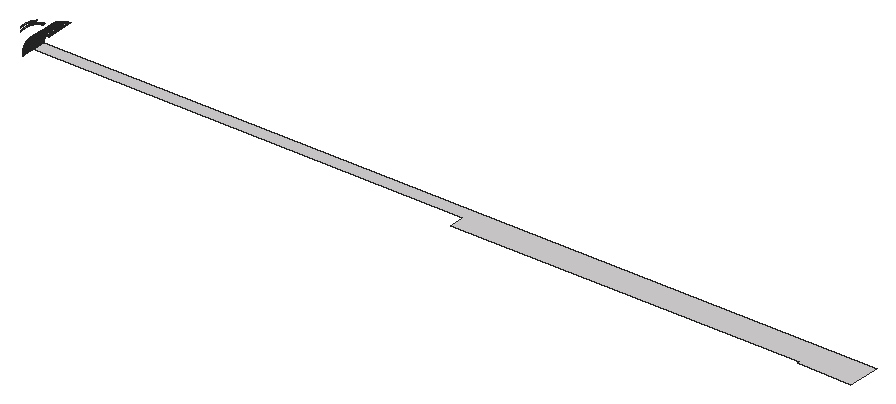
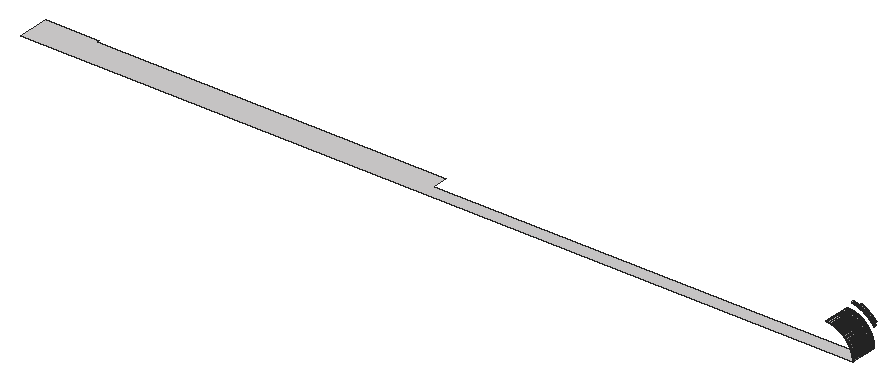
# SketchUp Ruby script. Lengths in inches.
U = 1.inch
M = Sketchup.active_model
def pt(a) = Geom::Point3d.new(a.map { |v| v * U })
def face(e, loops, mat)
  f = e.add_face(loops[0].map { |a| pt(a) })
  loops[1..].each { |l| e.add_face(l.map { |a| pt(a) }).erase! }
  f.material = f.back_material = mat if mat
  f
end
# faces: each face lists its corners as indices into pts; further lists are holes
def faces(e, pts, list, mat = nil) = list.each { |f| face(e, (f[0].is_a?(Array) ? f : [f]).map { |l| l.map { |i| pts[i] } }, mat) }
# xy, xz, yz: faces in a plane at the given z, y or x. An outline is a flat list of corners, or four numbers for a rectangle; further outlines are holes
def ring(l) = l.size == 4 ? [[l[0], l[1]], [l[2], l[1]], [l[2], l[3]], [l[0], l[3]]] : l.each_slice(2).to_a
def flat(e, list, mat, &to3) = list.each { |f| face(e, (f[0].is_a?(Array) ? f : [f]).map { |l| ring(l).map { |u, v| to3.(u, v) } }, mat) }
def xy(e, z, list, mat = nil) = flat(e, list, mat) { |x, y| [x, y, z] }
def xz(e, y, list, mat = nil) = flat(e, list, mat) { |x, z| [x, y, z] }
def yz(e, x, list, mat = nil) = flat(e, list, mat) { |y, z| [x, y, z] }
def lines(e, pts, list) = list.each { |a, b| e.add_line(pt(pts[a]), pt(pts[b])) }
# prism: a flat outline (further loops are holes) pulled along v
def prism(e, loops, v, mat = nil)
  f = face(e, loops, mat); d = Geom::Vector3d.new(v.map { |x| x * U })
  f.pushpull(f.normal.samedirection?(d) ? d.length : -d.length)
end
def box(e, o, s, mat = nil) = prism(e, [[o, [o[0] + s[0], o[1], o[2]], [o[0] + s[0], o[1] + s[1], o[2]], [o[0], o[1] + s[1], o[2]]]], [0, 0, s[2]], mat)
def at(x, y, z, deg = 0) = Geom::Transformation.translation(pt([x, y, z])) * Geom::Transformation.rotation(ORIGIN, Z_AXIS, deg.degrees)
def axes(o, x, y, z) = Geom::Transformation.new([*x, 0, *y, 0, *z, 0, *pt(o).to_a, 1])
def part(name) = M.definitions.add(name)
# library, detail: a bought-in or finely detailed component or shape, given as its bounding box
def library(name, o, s) = part(name).tap { |d| box(d.entities, o, s) }
def detail(e, o, s) = box(e.add_group.entities, o, s)
def put(e, d, t, mat = nil) = e.add_instance(d, t).tap { |i| i.material = mat if mat }
def group(e, t, mat = nil) = e.add_group.tap { |g| g.transformation = t; g.material = mat if mat }.entities
root = M.entities
M.materials.add("[Quartz Light Brown]").color = [215, 212, 212]
xy(root,84,[[372,36,396,36,396,50,24,50,24,44,216,44,216,37,372,37]],"[Quartz Light Brown]")
xy(root,95.96,[[34.96,38,35.06,50]],"[Quartz Light Brown]")
xy(root,95.98,[[35.25,38,35.34,50]],"[Quartz Light Brown]")
xy(root,95.99,[[35.43,38,35.53,50],[35.53,38,35.625,50]],"[Quartz Light Brown]")
xy(root,96,[[35.72,38,35.8125,50],[35.8125,38,35.91,50],[35.91,38,36,50]],"[Quartz Light Brown]")
yz(root,24,[[38,84,50,84.09],[38,84.09,50,84.1875],[38,84.1875,50,84.28]],"[Quartz Light Brown]")
yz(root,24.01,[[38,84.375,50,84.47],[38,84.47,50,84.57]],"[Quartz Light Brown]")
yz(root,24.02,[[38,84.66,50,84.75]],"[Quartz Light Brown]")
yz(root,24.04,[[38,84.94,50,85.04]],"[Quartz Light Brown]")
p = [[24.01,38,84.375],[24,38,84.28],[24,50,84.28],[24.01,50,84.375],[24.02,38,84.66],[24.01,38,84.57],
  [24.01,50,84.57],[24.02,50,84.66],[24.03,38,84.85],[24.02,38,84.75],[24.02,50,84.75],[24.03,50,84.85],
  [24.04,38,84.94],[24.04,50,84.94],[24.05,38,85.13],[24.04,38,85.04],[24.04,50,85.04],[24.05,50,85.13],
  [24.0625,38,85.22],[24.0625,50,85.22],[24.07,38,85.32],[24.07,50,85.32],[24.08,38,85.41],[24.08,50,85.41],
  [24.09,38,85.5],[24.09,50,85.5],[24.11,38,85.6],[24.11,50,85.6],[24.12,38,85.69],[24.12,50,85.69],
  [24.13,38,85.78],[24.13,50,85.78],[24.15,38,85.88],[24.15,50,85.88],[24.16,38,85.97],[24.16,50,85.97],
  [24.18,38,86.0625],[24.18,50,86.0625],[24.2,38,86.16],[24.2,50,86.16],[24.21,38,86.25],[24.21,50,86.25],
  [24.23,38,86.34],[24.23,50,86.34],[24.25,38,86.43],[24.25,50,86.43],[24.27,38,86.53],[24.27,50,86.53],
  [24.29,38,86.62],[24.29,50,86.62],[24.31,38,86.71],[24.31,50,86.71],[24.33,38,86.8],[24.33,50,86.8],
  [24.35,38,86.89],[24.35,50,86.89],[24.38,38,86.98],[24.38,50,86.98],[24.4,38,87.08],[24.4,50,87.08],
  [24.43,38,87.17],[24.43,50,87.17],[24.45,38,87.26],[24.45,50,87.26],[24.48,38,87.35],[24.48,50,87.35],
  [24.5,38,87.4375],[24.5,50,87.4375],[24.53,38,87.53],[24.53,50,87.53],[24.56,38,87.62],[24.56,50,87.62],
  [24.59,38,87.71],[24.59,50,87.71],[24.62,38,87.8],[24.62,50,87.8],[24.65,38,87.89],[24.65,50,87.89],
  [24.68,38,87.98],[24.68,50,87.98],[24.71,38,88.06],[24.71,50,88.06],[24.74,38,88.15],[24.74,50,88.15],
  [24.77,38,88.24],[24.77,50,88.24],[24.81,38,88.33],[24.81,50,88.33],[24.84,38,88.42],[24.84,50,88.42],
  [24.88,38,88.5],[24.88,50,88.5],[24.91,38,88.59],[24.91,50,88.59],[24.95,38,88.68],[24.95,50,88.68],
  [24.99,38,88.77],[24.99,50,88.77],[25.02,38,88.85],[25.02,50,88.85],[25.0625,38,88.9375],[25.0625,50,88.9375],
  [25.1,38,89.02],[25.1,50,89.02],[25.14,38,89.11],[25.14,50,89.11],[25.18,38,89.19],[25.18,50,89.19],
  [25.22,38,89.28],[25.22,50,89.28],[25.27,38,89.36],[25.27,50,89.36],[25.31,38,89.45],[25.31,50,89.45],
  [25.35,38,89.53],[25.35,50,89.53],[25.39,38,89.62],[25.39,50,89.62],[25.4375,38,89.7],[25.4375,50,89.7],
  [25.48,38,89.78],[25.48,50,89.78],[25.53,38,89.86],[25.53,50,89.86],[25.58,38,89.95],[25.58,50,89.95],
  [25.625,38,90.03],[25.625,50,90.03],[25.67,38,90.11],[25.67,50,90.11],[25.72,38,90.1875],[25.72,50,90.1875],
  [25.77,38,90.27],[25.77,50,90.27],[25.82,38,90.35],[25.82,50,90.35],[25.87,38,90.43],[25.87,50,90.43],
  [25.92,38,90.51],[25.92,50,90.51],[25.97,38,90.59],[25.97,50,90.59],[26.02,38,90.67],[26.02,50,90.67],
  [26.08,38,90.75],[26.08,50,90.75],[26.13,38,90.82],[26.13,50,90.82],[26.18,38,90.9],[26.18,50,90.9],
  [26.24,38,90.98],[26.24,50,90.98],[26.29,38,91.05],[26.29,50,91.05],[26.35,38,91.13],[26.35,50,91.13],
  [26.4,38,91.21],[26.4,50,91.21],[26.46,38,91.28],[26.46,50,91.28],[26.52,38,91.35],[26.52,50,91.35],
  [26.58,38,91.43],[26.58,50,91.43],[26.63,38,91.5],[26.63,50,91.5],[26.69,38,91.58],[26.69,50,91.58],
  [26.75,38,91.65],[26.75,50,91.65],[26.8125,38,91.72],[26.8125,50,91.72],[26.875,38,91.79],[26.875,50,91.79],
  [26.9375,38,91.86],[26.9375,50,91.86],[27,38,91.9375],[27,50,91.9375],[27.0625,38,92.01],[27.0625,50,92.01],
  [27.125,38,92.08],[27.125,50,92.08],[27.1875,38,92.15],[27.1875,50,92.15],[27.25,38,92.21],[27.25,50,92.21],
  [27.32,38,92.28],[27.32,50,92.28],[27.38,38,92.35],[27.38,50,92.35],[27.45,38,92.42],[27.45,50,92.42],
  [27.51,38,92.49],[27.51,50,92.49],[27.58,38,92.55],[27.58,50,92.55],[27.65,38,92.62],[27.65,50,92.62],
  [27.72,38,92.68],[27.72,50,92.68],[27.79,38,92.75],[27.79,50,92.75],[27.85,38,92.8125],[27.85,50,92.8125],
  [27.92,38,92.875],[27.92,50,92.875],[27.99,38,92.9375],[27.99,50,92.9375],[28.0625,38,93],[28.0625,50,93],
  [28.14,38,93.0625],[28.14,50,93.0625],[28.21,38,93.125],[28.21,50,93.125],[28.28,38,93.1875],[28.28,50,93.1875],
  [28.35,38,93.25],[28.35,50,93.25],[28.42,38,93.31],[28.42,50,93.31],[28.5,38,93.37],[28.5,50,93.37],
  [23.06,39,93.4],[23.06,38,93.4],[23.13,38,93.51],[23.13,39,93.51],[28.57,38,93.42],[28.57,50,93.42],
  [28.65,38,93.48],[28.65,50,93.48],[23.21,38,93.61],[23.21,39,93.61],[28.72,38,93.54],[28.72,50,93.54],
  [28.79,38,93.6],[28.79,50,93.6],[23.28,38,93.71],[23.28,39,93.71],[28.87,38,93.65],[28.87,50,93.65],
  [23.36,38,93.81],[23.36,39,93.81],[28.95,38,93.71],[28.95,50,93.71],[29.02,38,93.76],[29.02,50,93.76],
  [23.44,38,93.91],[23.44,39,93.91],[29.1,38,93.82],[29.1,50,93.82],[29.18,38,93.87],[29.18,50,93.87],
  [23.51,38,94],[23.51,39,94],[29.25,38,93.92],[29.25,50,93.92],[29.33,38,93.98],[29.33,50,93.98],
  [23.59,38,94.1],[23.59,39,94.1],[29.41,38,94.03],[29.41,50,94.03],[29.49,38,94.08],[29.49,50,94.08],
  [23.67,38,94.2],[23.67,39,94.2],[29.57,38,94.13],[29.57,50,94.13],[29.65,38,94.18],[29.65,50,94.18],
  [23.75,38,94.3],[23.75,39,94.3],[29.73,38,94.23],[29.73,50,94.23],[29.8125,38,94.28],[29.8125,50,94.28],
  [23.83,38,94.39],[23.83,39,94.39],[29.89,38,94.33],[29.89,50,94.33],[29.97,38,94.375],[29.97,50,94.375],
  [23.92,38,94.49],[23.92,39,94.49],[30.05,38,94.42],[30.05,50,94.42],[30.14,38,94.47],[30.14,50,94.47],
  [24,38,94.58],[24,39,94.58],[30.22,38,94.52],[30.22,50,94.52],[30.3,38,94.5625],[30.3,50,94.5625],
  [24.08,38,94.67],[24.08,39,94.67],[30.38,38,94.61],[30.38,50,94.61],[30.47,38,94.65],[30.47,50,94.65],
  [30.55,38,94.69],[30.55,50,94.69],[24.17,38,94.77],[24.17,39,94.77],[30.64,38,94.73],[30.64,50,94.73],
  [30.72,38,94.78],[30.72,50,94.78],[24.25,38,94.86],[24.25,39,94.86],[30.81,38,94.82],[30.81,50,94.82],
  [30.89,38,94.86],[30.89,50,94.86],[22.99,38,94.9375],[22.99,39,94.9375],[23.07,39,95.04],[23.07,38,95.04],
  [24.34,38,94.95],[24.34,39,94.95],[30.98,38,94.9],[30.98,50,94.9],[31.0625,38,94.9375],[31.0625,50,94.9375],
  [31.15,38,94.98],[31.15,50,94.98],[23.16,39,95.14],[23.16,38,95.14],[24.42,38,95.04],[24.42,39,95.04],
  [24.51,38,95.13],[24.51,39,95.13],[31.23,38,95.01],[31.23,50,95.01],[31.32,38,95.05],[31.32,50,95.05],
  [23.25,39,95.24],[23.25,38,95.24],[24.6,38,95.22],[24.6,39,95.22],[31.41,38,95.09],[31.41,50,95.09],
  [31.5,38,95.12],[31.5,50,95.12],[31.58,38,95.16],[31.58,50,95.16],[23.34,39,95.34],[23.34,38,95.34],
  [24.6875,38,95.3125],[24.6875,39,95.3125],[31.67,38,95.19],[31.67,50,95.19],[31.76,38,95.23],[31.76,50,95.23],
  [31.85,38,95.26],[31.85,50,95.26],[23.43,39,95.44],[23.43,38,95.44],[24.78,38,95.4],[24.78,39,95.4],
  [31.94,38,95.29],[31.94,50,95.29],[32.02,38,95.32],[32.02,50,95.32],[32.11,38,95.35],[32.11,50,95.35],
  [23.52,39,95.54],[23.52,38,95.54],[24.87,38,95.49],[24.87,39,95.49],[32.2,38,95.38],[32.2,50,95.38],
  [32.29,38,95.41],[32.29,50,95.41],[32.38,38,95.44],[32.38,50,95.44],[32.47,38,95.47],[32.47,50,95.47],
  [23.61,39,95.64],[23.61,38,95.64],[24.96,38,95.58],[24.96,39,95.58],[32.5625,38,95.5],[32.5625,50,95.5],
  [32.65,38,95.52],[32.65,50,95.52],[32.74,38,95.55],[32.74,50,95.55],[32.83,38,95.57],[32.83,50,95.57],
  [23.7,39,95.73],[23.7,38,95.73],[25.05,38,95.66],[25.05,39,95.66],[32.92,38,95.6],[32.92,50,95.6],
  [33.02,38,95.62],[33.02,50,95.62],[33.11,38,95.65],[33.11,50,95.65],[33.2,38,95.67],[33.2,50,95.67],
  [23.79,39,95.83],[23.79,38,95.83],[25.14,38,95.75],[25.14,39,95.75],[25.23,38,95.83],[25.23,39,95.83],
  [33.29,38,95.69],[33.29,50,95.69],[33.38,38,95.71],[33.38,50,95.71],[33.47,38,95.73],[33.47,50,95.73],
  [33.57,38,95.75],[33.57,50,95.75],[23.89,39,95.93],[23.89,38,95.93],[25.33,38,95.92],[25.33,39,95.92],
  [33.66,38,95.77],[33.66,50,95.77],[33.75,38,95.79],[33.75,50,95.79],[33.84,38,95.8],[33.84,50,95.8],
  [33.9375,38,95.82],[33.9375,50,95.82],[34.03,38,95.84],[34.03,50,95.84],[34.12,38,95.85],[34.12,50,95.85],
  [23.98,39,96.02],[23.98,38,96.02],[25.42,38,96],[25.42,39,96],[34.22,38,95.87],[34.22,50,95.87],
  [34.31,38,95.88],[34.31,50,95.88],[34.4,38,95.89],[34.4,50,95.89],[34.5,38,95.91],[34.5,50,95.91],
  [34.59,38,95.92],[34.59,50,95.92],[34.68,38,95.93],[34.68,50,95.93],[34.78,38,95.9375],[34.78,50,95.9375],
  [34.87,38,95.95],[34.87,50,95.95],[34.96,38,95.96],[34.96,50,95.96],[24.07,39,96.11],[24.07,38,96.11],
  [25.51,38,96.08],[25.51,39,96.08],[35.15,38,95.97],[35.06,38,95.96],[35.06,50,95.96],[35.15,50,95.97],
  [35.25,38,95.98],[35.25,50,95.98],[35.43,38,95.99],[35.34,38,95.98],[35.34,50,95.98],[35.43,50,95.99],
  [35.72,38,96],[35.625,38,95.99],[35.625,50,95.99],[35.72,50,96],[24.17,39,96.21],[24.17,38,96.21],
  [25.61,38,96.17],[25.61,39,96.17],[24.27,39,96.3],[24.27,38,96.3],[25.7,38,96.25],[25.7,39,96.25],
  [25.8,38,96.33],[25.8,39,96.33],[24.36,39,96.39],[24.36,38,96.39],[25.9,38,96.41],[25.9,39,96.41],
  [24.46,39,96.48],[24.46,38,96.48],[26,38,96.49],[26,39,96.49],[24.56,39,96.57],[24.56,38,96.57],
  [26.09,38,96.56],[26.09,39,96.56],[24.66,39,96.66],[24.66,38,96.66],[26.19,38,96.64],[26.19,39,96.64],
  [26.29,38,96.72],[26.29,39,96.72],[24.76,39,96.75],[24.76,38,96.75],[26.39,38,96.79],[26.39,39,96.79],
  [24.86,39,96.84],[24.86,38,96.84],[24.96,39,96.93],[24.96,38,96.93],[26.49,38,96.87],[26.49,39,96.87],
  [25.0625,39,97.01],[25.0625,38,97.01],[26.6,38,96.94],[26.6,39,96.94],[26.7,38,97.02],[26.7,39,97.02],
  [25.16,39,97.1],[25.16,38,97.1],[26.8,38,97.09],[26.8,39,97.09],[25.27,39,97.18],[25.27,38,97.18],
  [26.9,38,97.16],[26.9,39,97.16],[25.37,39,97.27],[25.37,38,97.27],[27.01,38,97.23],[27.01,39,97.23],
  [27.11,38,97.3],[27.11,39,97.3],[25.48,39,97.35],[25.48,38,97.35],[27.22,38,97.37],[27.22,39,97.37],
  [25.58,39,97.43],[25.58,38,97.43],[25.6875,39,97.51],[25.6875,38,97.51],[27.32,38,97.44],[27.32,39,97.44],
  [27.43,38,97.51],[27.43,39,97.51],[25.79,39,97.59],[25.79,38,97.59],[27.53,38,97.58],[27.53,39,97.58],
  [25.9,39,97.67],[25.9,38,97.67],[27.64,38,97.64],[27.64,39,97.64],[27.75,38,97.71],[27.75,39,97.71],
  [26.01,39,97.75],[26.01,38,97.75],[27.86,38,97.77],[27.86,39,97.77],[26.12,39,97.83],[26.12,38,97.83],
  [26.22,39,97.91],[26.22,38,97.91],[27.96,38,97.84],[27.96,39,97.84],[28.07,38,97.9],[28.07,39,97.9],
  [26.33,39,97.98],[26.33,38,97.98],[28.18,38,97.96],[28.18,39,97.96],[26.44,39,98.06],[26.44,38,98.06],
  [28.29,38,98.02],[28.29,39,98.02],[28.4,38,98.08],[28.4,39,98.08],[26.56,39,98.13],[26.56,38,98.13],
  [26.67,39,98.21],[26.67,38,98.21],[28.51,38,98.14],[28.51,39,98.14],[28.625,38,98.2],[28.625,39,98.2],
  [26.78,39,98.28],[26.78,38,98.28],[28.74,38,98.26],[28.74,39,98.26],[26.89,39,98.35],[26.89,38,98.35],
  [28.85,38,98.3125],[28.85,39,98.3125],[28.96,38,98.37],[28.96,39,98.37],[27,39,98.42],[27,38,98.42],
  [27.12,39,98.49],[27.12,38,98.49],[29.07,38,98.42],[29.07,39,98.42],[29.1875,38,98.48],[29.1875,39,98.48],
  [27.23,39,98.5625],[27.23,38,98.5625],[29.3,38,98.53],[29.3,39,98.53],[29.42,38,98.58],[29.42,39,98.58],
  [27.35,39,98.63],[27.35,38,98.63],[27.46,39,98.7],[27.46,38,98.7],[29.53,38,98.63],[29.53,39,98.63],
  [29.65,38,98.68],[29.65,39,98.68],[27.58,39,98.77],[27.58,38,98.77],[29.76,38,98.73],[29.76,39,98.73],
  [29.88,38,98.78],[29.88,39,98.78],[27.69,39,98.83],[27.69,38,98.83],[27.81,39,98.9],[27.81,38,98.9],
  [29.99,38,98.83],[29.99,39,98.83],[30.11,38,98.875],[30.11,39,98.875],[27.93,39,98.96],[27.93,38,98.96],
  [30.23,38,98.92],[30.23,39,98.92],[30.34,38,98.97],[30.34,39,98.97],[28.05,39,99.02],[28.05,38,99.02],
  [28.16,39,99.09],[28.16,38,99.09],[30.46,38,99.01],[30.46,39,99.01],[30.58,38,99.05],[30.58,39,99.05],
  [28.28,39,99.15],[28.28,38,99.15],[28.4,39,99.21],[28.4,38,99.21],[30.7,38,99.1],[30.7,39,99.1],
  [30.82,38,99.14],[30.82,39,99.14],[30.9375,38,99.18],[30.9375,39,99.18],[28.52,39,99.27],[28.52,38,99.27],
  [31.06,38,99.22],[31.06,39,99.22],[31.18,38,99.26],[31.18,39,99.26],[28.64,39,99.32],[28.64,38,99.32],
  [28.76,39,99.38],[28.76,38,99.38],[31.3,38,99.29],[31.3,39,99.29],[31.42,38,99.33],[31.42,39,99.33],
  [31.54,38,99.36],[31.54,39,99.36],[28.88,39,99.4375],[28.88,38,99.4375],[29,39,99.49],[29,38,99.49],
  [31.66,38,99.4],[31.66,39,99.4],[31.78,38,99.43],[31.78,39,99.43],[31.9,38,99.47],[31.9,39,99.47],
  [29.125,39,99.55],[29.125,38,99.55],[29.25,39,99.6],[29.25,38,99.6],[32.02,38,99.5],[32.02,39,99.5],
  [32.14,38,99.53],[32.14,39,99.53],[32.26,38,99.56],[32.26,39,99.56],[29.37,39,99.65],[29.37,38,99.65],
  [32.39,38,99.59],[32.39,39,99.59],[32.51,38,99.61],[32.51,39,99.61],[32.63,38,99.64],[32.63,39,99.64],
  [32.76,38,99.67],[32.76,39,99.67],[29.49,39,99.71],[29.49,38,99.71],[29.62,39,99.76],[29.62,38,99.76],
  [32.88,38,99.69],[32.88,39,99.69],[33,38,99.72],[33,39,99.72],[33.125,38,99.74],[33.125,39,99.74],
  [33.25,38,99.76],[33.25,39,99.76],[29.74,39,99.81],[29.74,38,99.81]]
faces(root,p,[[0,1,2,3],[4,5,6,7],[8,9,10,11],[12,8,11,13],[14,15,16,17],[18,14,17,19],[20,18,19,21],[22,20,21,23],
  [24,22,23,25],[26,24,25,27],[28,26,27,29],[30,28,29,31],[32,30,31,33],[34,32,33,35],[36,34,35,37],[38,36,37,39],
  [40,38,39,41],[42,40,41,43],[44,42,43,45],[46,44,45,47],[48,46,47,49],[50,48,49,51],[52,50,51,53],[54,52,53,55],
  [56,54,55,57],[58,56,57,59],[60,58,59,61],[62,60,61,63],[64,62,63,65],[66,64,65,67],[68,66,67,69],[70,68,69,71],
  [72,70,71,73],[74,72,73,75],[76,74,75,77],[78,76,77,79],[80,78,79,81],[82,80,81,83],[84,82,83,85],[86,84,85,87],
  [88,86,87,89],[90,88,89,91],[92,90,91,93],[94,92,93,95],[96,94,95,97],[98,96,97,99],[100,98,99,101],[102,100,101,103],
  [104,102,103,105],[106,104,105,107],[108,106,107,109],[110,108,109,111],[112,110,111,113],[114,112,113,115],[116,114,115,117],[118,116,117,119],
  [120,118,119,121],[122,120,121,123],[124,122,123,125],[126,124,125,127],[128,126,127,129],[130,128,129,131],[132,130,131,133],[134,132,133,135],
  [136,134,135,137],[138,136,137,139],[140,138,139,141],[142,140,141,143],[144,142,143,145],[146,144,145,147],[148,146,147,149],[150,148,149,151],
  [152,150,151,153],[154,152,153,155],[156,154,155,157],[158,156,157,159],[160,158,159,161],[162,160,161,163],[164,162,163,165],[166,164,165,167],
  [168,166,167,169],[170,168,169,171],[172,170,171,173],[174,172,173,175],[176,174,175,177],[178,176,177,179],[180,178,179,181],[182,180,181,183],
  [184,182,183,185],[186,184,185,187],[188,186,187,189],[190,188,189,191],[192,190,191,193],[194,192,193,195],[196,194,195,197],[198,196,197,199],
  [200,198,199,201],[202,200,201,203],[204,202,203,205],[206,204,205,207],[208,206,207,209],[210,208,209,211],[212,210,211,213],[214,212,213,215],
  [216,214,215,217],[218,216,217,219],[220,218,219,221],[222,223,224,225],[226,220,221,227],[228,226,227,229],[225,224,230,231],[232,228,229,233],
  [234,232,233,235],[231,230,236,237],[238,234,235,239],[237,236,240,241],[242,238,239,243],[244,242,243,245],[241,240,246,247],[248,244,245,249],
  [250,248,249,251],[247,246,252,253],[254,250,251,255],[256,254,255,257],[253,252,258,259],[260,256,257,261],[262,260,261,263],[259,258,264,265],
  [266,262,263,267],[268,266,267,269],[265,264,270,271],[272,268,269,273],[274,272,273,275],[271,270,276,277],[278,274,275,279],[280,278,279,281],
  [277,276,282,283],[284,280,281,285],[286,284,285,287],[283,282,288,289],[290,286,287,291],[292,290,291,293],[289,288,294,295],[296,292,293,297],
  [298,296,297,299],[300,298,299,301],[295,294,302,303],[304,300,301,305],[306,304,305,307],[303,302,308,309],[310,306,307,311],[312,310,311,313],
  [314,315,316,317],[309,308,318,319],[320,312,313,321],[322,320,321,323],[324,322,323,325],[317,316,326,327],[319,318,328,329],[329,328,330,331],
  [332,324,325,333],[334,332,333,335],[327,326,336,337],[331,330,338,339],[340,334,335,341],[342,340,341,343],[344,342,343,345],[337,336,346,347],
  [339,338,348,349],[350,344,345,351],[352,350,351,353],[354,352,353,355],[347,346,356,357],[349,348,358,359],[360,354,355,361],[362,360,361,363],
  [364,362,363,365],[357,356,366,367],[359,358,368,369],[370,364,365,371],[372,370,371,373],[374,372,373,375],[376,374,375,377],[367,366,378,379],
  [369,368,380,381],[382,376,377,383],[384,382,383,385],[386,384,385,387],[388,386,387,389],[379,378,390,391],[381,380,392,393],[394,388,389,395],
  [396,394,395,397],[398,396,397,399],[400,398,399,401],[391,390,402,403],[393,392,404,405],[405,404,406,407],[408,400,401,409],[410,408,409,411],
  [412,410,411,413],[414,412,413,415],[403,402,416,417],[407,406,418,419],[420,414,415,421],[422,420,421,423],[424,422,423,425],[426,424,425,427],
  [428,426,427,429],[430,428,429,431],[417,416,432,433],[419,418,434,435],[436,430,431,437],[438,436,437,439],[440,438,439,441],[442,440,441,443],
  [444,442,443,445],[446,444,445,447],[448,446,447,449],[450,448,449,451],[452,450,451,453],[433,432,454,455],[435,434,456,457],[458,459,460,461],
  [462,458,461,463],[464,465,466,467],[468,469,470,471],[455,454,472,473],[457,456,474,475],[473,472,476,477],[475,474,478,479],[479,478,480,481],
  [477,476,482,483],[481,480,484,485],[483,482,486,487],[485,484,488,489],[487,486,490,491],[489,488,492,493],[491,490,494,495],[493,492,496,497],
  [497,496,498,499],[495,494,500,501],[499,498,502,503],[501,500,504,505],[505,504,506,507],[503,502,508,509],[507,506,510,511],[509,508,512,513],
  [513,512,514,515],[511,510,516,517],[515,514,518,519],[517,516,520,521],[519,518,522,523],[521,520,524,525],[523,522,526,527],[527,526,528,529],
  [525,524,530,531],[529,528,532,533],[531,530,534,535],[535,534,536,537],[533,532,538,539],[539,538,540,541],[537,536,542,543],[541,540,544,545],
  [543,542,546,547],[545,544,548,549],[549,548,550,551],[547,546,552,553],[551,550,554,555],[553,552,556,557],[557,556,558,559],[555,554,560,561],
  [561,560,562,563],[559,558,564,565],[563,562,566,567],[565,564,568,569],[567,566,570,571],[571,570,572,573],[569,568,574,575],[575,574,576,577],
  [573,572,578,579],[579,578,580,581],[577,576,582,583],[581,580,584,585],[583,582,586,587],[585,584,588,589],[589,588,590,591],[587,586,592,593],
  [593,592,594,595],[591,590,596,597],[597,596,598,599],[595,594,600,601],[599,598,602,603],[603,602,604,605],[601,600,606,607],[607,606,608,609],
  [605,604,610,611],[611,610,612,613],[609,608,614,615],[613,612,616,617],[617,616,618,619],[615,614,620,621],[621,620,622,623],[619,618,624,625],
  [625,624,626,627],[623,622,628,629],[627,626,630,631],[631,630,632,633],[629,628,634,635],[635,634,636,637],[633,632,638,639],[639,638,640,641],
  [637,636,642,643],[643,642,644,645],[641,640,646,647],[647,646,648,649],[649,648,650,651],[645,644,652,653],[651,650,654,655],[655,654,656,657],
  [653,652,658,659],[659,658,660,661],[657,656,662,663],[663,662,664,665],[665,664,666,667],[661,660,668,669],[669,668,670,671],[667,666,672,673],
  [673,672,674,675],[675,674,676,677],[671,670,678,679],[679,678,680,681],[677,676,682,683],[683,682,684,685],[685,684,686,687],[681,680,688,689],
  [687,686,690,691],[691,690,692,693],[693,692,694,695],[695,694,696,697],[689,688,698,699],[699,698,700,701],[697,696,702,703],[703,702,704,705],
  [705,704,706,707],[707,706,708,709],[701,700,710,711]],"[Quartz Light Brown]")
